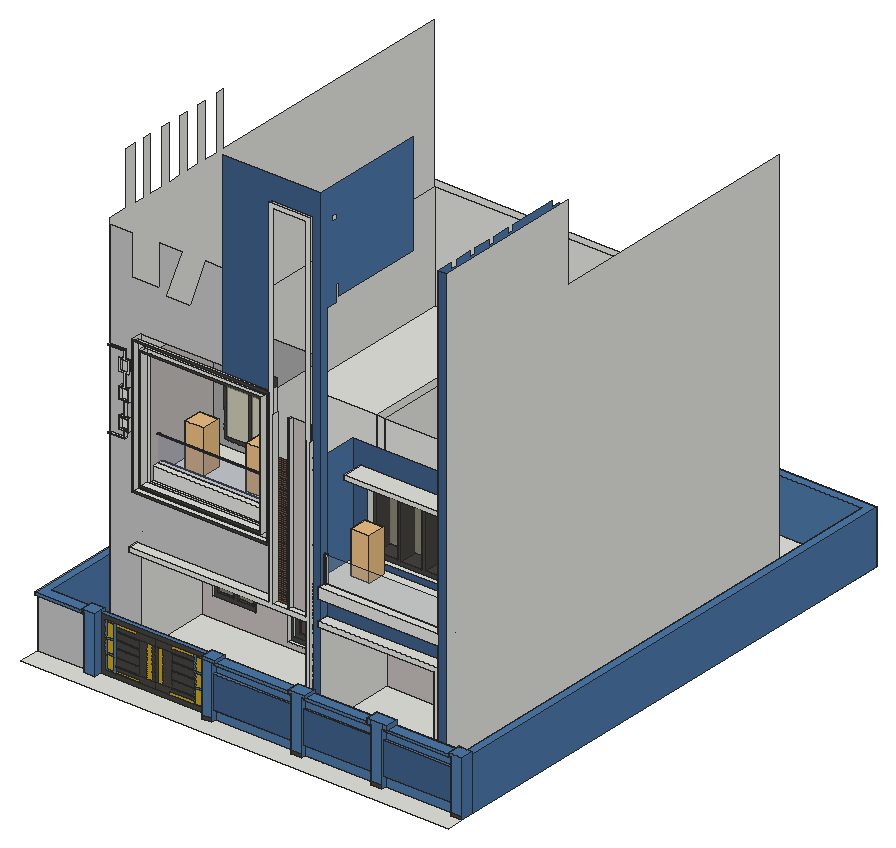
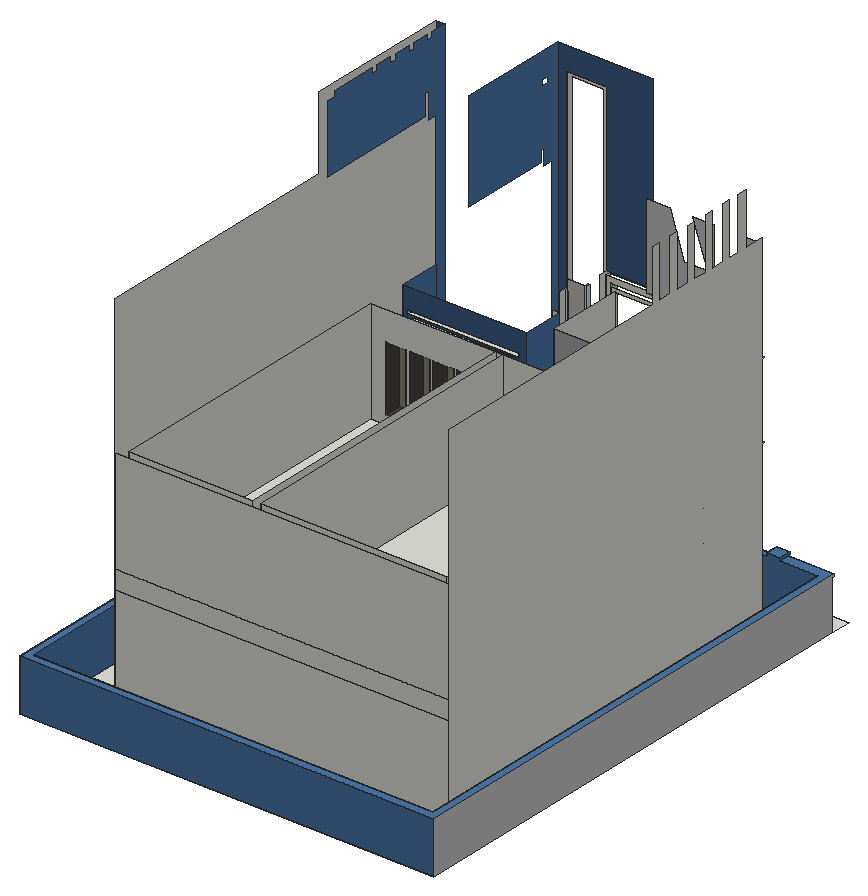
# SketchUp Ruby script. Lengths in inches.
U = 1.inch
M = Sketchup.active_model
def pt(a) = Geom::Point3d.new(a.map { |v| v * U })
def face(e, loops, mat)
  f = e.add_face(loops[0].map { |a| pt(a) })
  loops[1..].each { |l| e.add_face(l.map { |a| pt(a) }).erase! }
  f.material = f.back_material = mat if mat
  f
end
# faces: each face lists its corners as indices into pts; further lists are holes
def faces(e, pts, list, mat = nil) = list.each { |f| face(e, (f[0].is_a?(Array) ? f : [f]).map { |l| l.map { |i| pts[i] } }, mat) }
# xy, xz, yz: faces in a plane at the given z, y or x. An outline is a flat list of corners, or four numbers for a rectangle; further outlines are holes
def ring(l) = l.size == 4 ? [[l[0], l[1]], [l[2], l[1]], [l[2], l[3]], [l[0], l[3]]] : l.each_slice(2).to_a
def flat(e, list, mat, &to3) = list.each { |f| face(e, (f[0].is_a?(Array) ? f : [f]).map { |l| ring(l).map { |u, v| to3.(u, v) } }, mat) }
def xy(e, z, list, mat = nil) = flat(e, list, mat) { |x, y| [x, y, z] }
def xz(e, y, list, mat = nil) = flat(e, list, mat) { |x, z| [x, y, z] }
def yz(e, x, list, mat = nil) = flat(e, list, mat) { |y, z| [x, y, z] }
def lines(e, pts, list) = list.each { |a, b| e.add_line(pt(pts[a]), pt(pts[b])) }
# prism: a flat outline (further loops are holes) pulled along v
def prism(e, loops, v, mat = nil)
  f = face(e, loops, mat); d = Geom::Vector3d.new(v.map { |x| x * U })
  f.pushpull(f.normal.samedirection?(d) ? d.length : -d.length)
end
def box(e, o, s, mat = nil) = prism(e, [[o, [o[0] + s[0], o[1], o[2]], [o[0] + s[0], o[1] + s[1], o[2]], [o[0], o[1] + s[1], o[2]]]], [0, 0, s[2]], mat)
def at(x, y, z, deg = 0) = Geom::Transformation.translation(pt([x, y, z])) * Geom::Transformation.rotation(ORIGIN, Z_AXIS, deg.degrees)
def axes(o, x, y, z) = Geom::Transformation.new([*x, 0, *y, 0, *z, 0, *pt(o).to_a, 1])
def part(name) = M.definitions.add(name)
# library, detail: a bought-in or finely detailed component or shape, given as its bounding box
def library(name, o, s) = part(name).tap { |d| box(d.entities, o, s) }
def detail(e, o, s) = box(e.add_group.entities, o, s)
def put(e, d, t, mat = nil) = e.add_instance(d, t).tap { |i| i.material = mat if mat }
def group(e, t, mat = nil) = e.add_group.tap { |g| g.transformation = t; g.material = mat if mat }.entities
root = M.entities
M.materials.add("!长灌木1").color = [90, 107, 61]
M.materials.add("Brick_09_1K").color = [77, 120, 168]
M.materials.add("Brick_09_1K1").color = [62, 96, 135]
M.materials.add("Glass_Basic_01").color = [161, 173, 186]
M.materials["Glass_Basic_01"].alpha = 0.25
M.materials.add("Glass_Mirror_01").color = [188, 186, 154]
M.materials["Glass_Mirror_01"].alpha = 0.57
M.materials.add("Glass_Sky Reflection_01").color = [126, 138, 183]
M.materials["Glass_Sky Reflection_01"].alpha = 0.25
M.materials.add("Image3").color = [196, 190, 186]
M.materials.add("M02_Ash_Whisper").color = [196, 196, 196]
M.materials.add("M03_Pewter_Shine").color = [168, 168, 168]
M.materials.add("Material20").color = [184, 138, 65]
M.materials.add("Material48").color = [126, 124, 110]
M.materials.add("Metal_32_1K").color = [117, 124, 125]
M.materials.add("Metal_Perforated_08_1K").color = [201, 163, 22]
M.materials.add("Wood_Floor_12_1K").color = [92, 75, 65]
M.materials.add("Wood_Planks_01_1K").color = [69, 67, 63]
M.materials.add("Wood_Veneer_15_1K").color = [132, 88, 57]
c1 = part("组\#1")
xy(c1.entities,0,[[0,0,2.36,2.36],[29.92,0,32.28,2.36],[0,29.92,2.36,32.28],[29.92,29.92,32.28,32.28]],"Material48")
xy(c1.entities,1.57,[[2.36,0.39,2.36,2.36,0.39,2.36,0.39,29.92,2.36,29.92,2.36,31.89,29.92,31.89,29.92,29.92,31.89,29.92,31.89,2.36,29.92,2.36,29.92,0.39]],"Material48")
xy(c1.entities,2.76,[[3.54,0.39,28.74,1.57],[0.39,3.54,1.57,28.74],[30.71,3.54,31.89,28.74],[3.54,30.71,28.74,31.89]],"Material20")
xy(c1.entities,20.08,[[3.54,0.39,28.74,1.57],[0.39,3.54,1.57,28.74],[30.71,3.54,31.89,28.74],[3.54,30.71,28.74,31.89]],"Material20")
xy(c1.entities,21.0625,[[2.36,2.36,29.92,29.92]],"!长灌木1")
xy(c1.entities,21.26,[[2.36,0.39,29.92,2.36],[0.39,2.36,2.36,29.92],[29.92,2.36,31.89,29.92],[2.36,29.92,29.92,31.89]],"Material20")
xy(c1.entities,21.38,[[2.36,2.36,29.92,29.92]],"!长灌木1")
xy(c1.entities,22.83,[[0,0,2.36,2.36],[29.92,0,32.28,2.36],[0,29.92,2.36,32.28],[29.92,29.92,32.28,32.28]],"Material20")
xz(c1.entities,0,[[0,0,2.36,22.83],[29.92,0,32.28,22.83]],"Material20")
xz(c1.entities,0.39,[[[2.36,1.57,29.92,21.26],[3.54,2.76,28.74,20.08]]],"Material20")
xz(c1.entities,1.57,[[3.54,2.76,28.74,20.08]],"Material20")
xz(c1.entities,2.36,[[2.36,21.0625,29.92,21.38],[2.36,21.26,29.92,23.43]],"!长灌木1")
xz(c1.entities,2.36,[[0,0,0,22.83,2.36,22.83,2.36,21.26,0.39,21.26,0.39,1.57,2.36,1.57,2.36,0],[29.92,0,29.92,1.57,31.89,1.57,31.89,21.26,29.92,21.26,29.92,22.83,32.28,22.83,32.28,0]],"Material20")
xz(c1.entities,3.54,[[0.39,2.76,1.57,20.08],[30.71,2.76,31.89,20.08]],"Material20")
xz(c1.entities,28.74,[[0.39,2.76,1.57,20.08],[30.71,2.76,31.89,20.08]],"Material20")
xz(c1.entities,29.92,[[2.36,21.0625,29.92,21.38],[2.36,21.26,29.92,23.43]],"!长灌木1")
xz(c1.entities,29.92,[[0,0,2.36,0,2.36,1.57,0.39,1.57,0.39,22.83,0,22.83],[29.92,0,32.28,0,32.28,22.83,31.89,22.83,31.89,1.57,29.92,1.57],[0.39,21.26,2.36,22.83],[29.92,21.26,31.89,22.83]],"Material20")
xz(c1.entities,30.71,[[3.54,2.76,28.74,20.08]],"Material20")
xz(c1.entities,31.89,[[[2.36,1.57,29.92,21.26],[3.54,2.76,28.74,20.08]]],"Material20")
xz(c1.entities,32.28,[[0,0,2.36,22.83],[29.92,0,32.28,22.83]],"Material20")
yz(c1.entities,0,[[0,0,2.36,22.83],[29.92,0,32.28,22.83]],"Material20")
yz(c1.entities,0.39,[[[2.36,1.57,29.92,21.26],[3.54,2.76,28.74,20.08]]],"Material20")
yz(c1.entities,1.57,[[3.54,2.76,28.74,20.08]],"Material20")
yz(c1.entities,2.36,[[0,0,2.36,0,2.36,1.57,0.39,1.57,0.39,22.83,0,22.83]])
yz(c1.entities,2.36,[[2.36,21.0625,29.92,21.38],[2.36,21.26,29.92,23.43]],"!长灌木1")
yz(c1.entities,2.36,[[29.92,0,32.28,0,32.28,22.83,29.92,22.83,29.92,21.26,31.89,21.26,31.89,1.57,29.92,1.57],[0.39,21.26,2.36,22.83]],"Material20")
yz(c1.entities,3.54,[[0.39,2.76,1.57,20.08],[30.71,2.76,31.89,20.08]],"Material20")
yz(c1.entities,28.74,[[0.39,2.76,1.57,20.08],[30.71,2.76,31.89,20.08]],"Material20")
yz(c1.entities,29.92,[[2.36,21.0625,29.92,21.38],[2.36,21.26,29.92,23.43]],"!长灌木1")
yz(c1.entities,29.92,[[0,0,0,22.83,2.36,22.83,2.36,21.26,0.39,21.26,0.39,1.57,2.36,1.57,2.36,0],[29.92,0,29.92,1.57,31.89,1.57,31.89,21.26,29.92,21.26,29.92,22.83,32.28,22.83,32.28,0]],"Material20")
yz(c1.entities,30.71,[[3.54,2.76,28.74,20.08]],"Material20")
yz(c1.entities,31.89,[[[2.36,1.57,29.92,21.26],[3.54,2.76,28.74,20.08]]],"Material20")
yz(c1.entities,32.28,[[0,0,2.36,22.83],[29.92,0,32.28,22.83]],"Material20")
c2 = part("组\#2")
put(c2.entities,c1,at(24.1,23.99,0))
c3 = part("Potted tree")
put(c3.entities,c2,at(-24.1,-23.99,-1.57))
c4 = library("Group_2",[-1.28,-0.39,0],[21.22,20.51,48.44])
xy(root,0,[[0,0,480,0,480,19,468,19,468,24,390.18,24,390.18,19,378.18,19,378.18,24,300.36,24,300.36,19,288.36,19,288.36,24,199.54,24,199.54,19,188.41,19,188.41,27.57,68.53,27.57,68.53,19,56.53,19,56.53,24,0,24],[[56.53,19,68.53,19,68.53,27.57,188.41,27.57,188.41,19,199.54,19,199.54,24,288.36,24,288.36,19,300.36,19,300.36,24,378.18,24,378.18,19,390.18,19,390.18,24,468,24,468,19,480,19,480,600,0,600,0,24,56.53,24],[9,33,471,591]],[[9,33,471,591],[265,69,265,81,270,81,270,165,71.88,165,71.88,81,36,81,36,534,423,534,423,69,408.87,69,408.87,165,279,165,279,72.06,270,72.06,270,69]],[413,69,423,165],[270,72.06,279,165],
  [36,81,71.88,165],[45,174,261,525],[270,174,414,525]])
xy(root,6,[[168,165,240,168.66]])
xy(root,10,[[172,168.66,204,170.16],[204,168.66,236,170.99]])
xy(root,12,[[199.54,21,288.36,24],[300.36,21,378.18,24],[390.18,21,468,24]],"Brick_09_1K")
xy(root,15,[[177,170.16,199,172.08],[209,170.99,231,172.5],[177,172.08,199,174],[209,172.5,231,174]],"Wood_Planks_01_1K")
xy(root,21.3,[[341,165,401,167.38]])
xy(root,21.88,[[84,165,132,166.72]])
xy(root,25.3,[[345,167.38,369,167.38,373,167.86,373,170.69,345,170.69],[373,167.38,397,167.38,397,170.69,373,167.86],[373,167.86,397,170.69,373,170.69],[345,170.69,373,170.69,373,173.53,369,174,345,174],[373,170.69,397,170.69,373,173.53],
  [397,170.69,397,174,373,174,373,173.53]],"Wood_Planks_01_1K")
xy(root,25.88,[[88,166.72,106,170.36],[110,166.72,128,170.36],[88,170.36,106,174],[110,170.36,128,174]],"Wood_Planks_01_1K")
xy(root,48,[[199.54,21,288.36,24],[300.36,21,378.18,24],[390.18,21,468,24]],"Brick_09_1K")
xy(root,57,[[0,21,56.53,24],[199.54,21,288.36,24],[300.36,21,378.18,24],[390.18,21,468,24]],"Brick_09_1K")
xy(root,60,[[53.53,19,56.53,21],[199.54,19,202.54,21],[285.36,19,288.36,21],[300.36,19,303.36,21],[373.51,19,378.18,21],
  [390.18,19,395.5625,21],[465,19,468,21],[0,21,53.53,21,53.53,33,9,33,9,591,471,591,471,33,480,33,480,600,0,600],[202.54,21,285.36,33],[303.36,21,373.51,33],
  [395.5625,21,465,33],[68.53,27.57,188.41,33]],"Brick_09_1K")
xy(root,63,[[53.53,19,68.53,33],[188.41,19,202.54,33],[285.36,19,303.36,33],[465,19,480,33]],"Brick_09_1K")
xy(root,65.38,[[373.51,19,395.5625,33]],"Brick_09_1K")
xy(root,81,[[177,170.16,199,172.08],[209,170.99,231,172.5],[177,172.08,199,174],[209,172.5,231,174]],"Wood_Planks_01_1K")
xy(root,86,[[172,168.66,204,170.16],[204,168.66,236,170.99]])
xy(root,86,[[88,166.72,106,170.36],[110,166.72,128,170.36],[345,167.38,345,170.69,373,170.69,373,167.86,369,167.38],[373,167.38,373,167.86,397,170.69,397,167.38],[373,167.86,373,170.69,397,170.69],
  [88,170.36,106,174],[110,170.36,128,174],[345,170.69,345,174,369,174,373,173.53,373,170.69],[373,170.69,373,173.53,397,170.69],[397,170.69,373,173.53,373,174,397,174]],"Wood_Planks_01_1K")
xy(root,90,[[84,165,132,166.72],[168,165,240,168.66],[341,165,401,167.38]])
xy(root,102,[[66.12,69,71.88,81],[71.88,69,71.88,165,261,165,261,81,223.07,81,223.07,69],[223.07,69,265,81],[279,69,408.87,165],[261,81,270,165],
  [270,81,279,165]])
xy(root,107,[[66.12,69,223.07,81],[228.07,69,265,69,265,75.9,244.4,75.9,244.4,72.3125,242.32,72.3125,242.32,75.9,228.07,75.9]])
xy(root,108,[[279,69,413,81]])
xy(root,130,[[279,69,413,81]])
xy(root,142,[[279,69,413,69,413,77.38,282.2,77.38,282.2,76.04,279,76.04],[282.2,77.38,413,77.38,413,129,270,129,270,81,279,81,279,78.72,282.2,78.72],[261,81,270,165],[45,174,261,525],[270,174,414,525]])
xy(root,148,[[287,129,401,135.39]])
xy(root,152,[[291,135.39,314.5,154.7],[318.5,135.39,342,174],[346,135.39,369.5,174],[373.5,135.39,397,174],[291,154.7,314.5,174]],"Wood_Planks_01_1K")
xy(root,164,[[70,69,223.07,81]])
xy(root,166,[[72,69,221.07,75]])
xy(root,172,[[78,69,215.07,75],[279,76.04,282.2,78.72]])
xy(root,174,[[80,69,213.07,77.68]])
xy(root,175.72,[[84,77.68,209.07,81]])
xy(root,178,[[84,93.35,209.07,165]])
xy(root,190,[[84,81,209.07,81,209.07,87.18,84,87.26],[209.07,87.18,209.07,93.35,84,93.35,84,87.26]])
xy(root,207.65,[[36,78,55,81]])
xy(root,208.65,[[36,78,54,81]])
xy(root,215.87,[[48.51,78,54,81],[55,78,59.4,81]])
xy(root,216.87,[[49.51,78,58.4,81]])
xy(root,228,[[291,135.39,314.5,154.7],[318.5,135.39,342,174],[346,135.39,369.5,174],[373.5,135.39,397,174],[291,154.7,314.5,174]],"Wood_Planks_01_1K")
xy(root,228.74,[[49.51,78,58.4,81]])
xy(root,229.74,[[48.51,78,54,81],[55,78,59.4,81]])
xy(root,232,[[287,129,401,135.39]])
xy(root,233.78,[[279.03,105,407.71,129]])
xy(root,238.38,[[279.03,105,407.71,129]])
xy(root,245.55,[[48.51,78,54,81],[55,78,59.4,81]])
xy(root,246.55,[[49.51,78,58.4,81]])
xz(root,19,[[56.53,0,68.53,63],[188.41,4,199.54,60],[288.36,4,300.36,4,300.36,60,303.36,60,303.36,63,285.36,63,285.36,60,288.36,60],[378.18,4,390.18,65.38],[468,4,480,4,480,63,465,63,465,60,468,60],
  [53.53,60,56.53,63],[188.41,60,202.54,63],[373.51,60,378.18,65.38],[390.18,60,395.5625,65.38]],"Brick_09_1K")
xz(root,19,[[188.41,0,199.54,4],[288.36,0,300.36,4],[378.18,0,390.18,4],[468,0,480,4]],"Wood_Planks_01_1K")
xz(root,21,[[0,57,56.53,60],[199.54,57,288.36,60],[300.36,57,378.18,60],[390.18,57,468,60]],"Brick_09_1K")
xz(root,21,[[199.54,12,288.36,48],[300.36,12,378.18,48],[390.18,12,468,48]],"Brick_09_1K1")
xz(root,24,[[199.54,0,288.36,12],[300.36,0,378.18,12],[390.18,0,468,12],[199.54,48,288.36,57],[300.36,48,378.18,57],
  [390.18,48,468,57]],"Brick_09_1K")
xz(root,24,[[0,0,56.53,57]],"M02_Ash_Whisper")
xz(root,27.57,[[[72.53,4,84.53,56],[74.53,6,82.53,54]],[[172.41,4,184.41,56],[174.41,6,182.41,54]],[84.53,12,110.66,13],[147.49,12,172.41,13],[84.53,20.75,110.66,21.75],
  [147.49,20.75,172.41,21.75],[74.53,21.33,82.53,23.33],[174.41,21.33,182.41,23.33],[84.53,29.5,110.66,30.5],[147.49,29.5,172.41,30.5],
  [74.53,36.67,82.53,38.67],[174.41,36.67,182.41,38.67],[84.53,38.25,110.66,39.25],[147.49,38.25,172.41,39.25],[84.53,47,110.66,48],
  [147.49,47,172.41,48]],"Brick_09_1K")
xz(root,27.57,[[84.53,5.11,111.61,8],[145.17,5.11,172.41,8],[74.53,6,82.53,21.33],[174.41,6,182.41,21.33],[119.57,12,125.31,48],
  [131.65,12,137.98,48],[74.53,23.33,82.53,36.67],[174.41,23.33,182.41,36.67],[74.53,38.67,82.53,54],[174.41,38.67,182.41,54],
  [84.53,52,108.53,56],[148.41,52,172.41,56]],"Metal_Perforated_08_1K")
xz(root,27.57,[[[68.53,0,188.41,60],[72.53,4,184.41,56]],[84.53,4,128.47,4,128.47,12,84.53,12,84.53,8,111.61,8,111.61,5.11,84.53,5.11],[128.47,4,172.41,4,172.41,5.11,145.17,5.11,145.17,8,172.41,8,172.41,12,128.47,12],[110.66,12,119.57,48],[125.31,12,128.47,48],
  [128.47,12,131.65,48],[137.98,12,147.49,48],[84.53,13,110.66,20.75],[147.49,13,172.41,20.75],[84.53,21.75,110.66,29.5],
  [147.49,21.75,172.41,29.5],[84.53,30.5,110.66,38.25],[147.49,30.5,172.41,38.25],[84.53,39.25,110.66,47],[147.49,39.25,172.41,47],
  [84.53,48,128.47,48,128.47,56,108.53,56,108.53,52,84.53,52],[128.47,48,172.41,48,172.41,52,148.41,52,148.41,56,128.47,56]],"Wood_Planks_01_1K")
xz(root,33,[[9,0,9,60,53.53,60,53.53,63,68.53,63,68.53,60,188.41,60,188.41,63,202.54,63,202.54,60,285.36,60,285.36,63,303.36,63,303.36,60,373.51,60,373.51,65.38,395.5625,65.38,395.5625,60,465,60,465,63,471,63,471,0],[471,60,480,63]],"Brick_09_1K")
xz(root,69,[[[265,0,270,0,270,509.43,223.07,509.43,223.07,107,66.12,107,66.12,102,265,102],[228.07,107,265,504.43]],[408.87,0,413,0,413,108,279,108,279,102,408.87,102],[279,130,413,142]])
xz(root,69,[[413,0,423,506.58]],"Brick_09_1K1")
xz(root,69,[[[70,164,223.07,318],[72,166,221.07,316]],[[78,172,215.07,310],[80,174,213.07,308]]],"Wood_Planks_01_1K")
xz(root,72.06,[[270,0,279,0,279,536.58,169.4,536.58,169.4,318,223.07,318,223.07,509.43,270,509.43]],"Brick_09_1K1")
xz(root,72.3125,[[242.32,107,244.4,297.09]])
xz(root,75,[[[72,166,221.07,316],[78,172,215.07,310]]])
xz(root,75.9,[[244.4,107,265,297.09]],"Image3")
xz(root,75.9,[[228.07,107,242.32,108.9],[228.07,108.9,242.32,110.8],[228.07,110.8,242.32,112.7],[228.07,112.7,242.32,114.6],[228.07,114.6,242.32,116.5],
  [228.07,116.5,242.32,118.41],[228.07,118.41,242.32,120.31],[228.07,120.31,242.32,122.21],[228.07,122.21,242.32,124.11],[228.07,124.11,242.32,126.01],
  [228.07,126.01,242.32,127.91],[228.07,127.91,242.32,129.8125],[228.07,129.8125,242.32,131.71],[228.07,131.71,242.32,133.61],[228.07,133.61,242.32,135.51],
  [228.07,135.51,242.32,137.42],[228.07,137.42,242.32,139.32],[228.07,139.32,242.32,141.22],[228.07,141.22,242.32,143.12],[228.07,143.12,242.32,145.02],
  [228.07,145.02,242.32,146.92],[228.07,146.92,242.32,148.82],[228.07,148.82,242.32,150.72],[228.07,150.72,242.32,152.62],[228.07,152.62,242.32,154.52],
  [228.07,154.52,242.32,156.42],[228.07,156.42,242.32,158.33],[228.07,158.33,242.32,160.23],[228.07,160.23,242.32,162.13],[228.07,162.13,242.32,164.03],
  [228.07,164.03,242.32,165.93],[228.07,165.93,242.32,167.83],[228.07,167.83,242.32,169.73],[228.07,169.73,242.32,171.63],[228.07,171.63,242.32,173.53],
  [228.07,173.53,242.32,175.43],[228.07,175.43,242.32,177.33],[228.07,177.33,242.32,179.24],[228.07,179.24,242.32,181.14],[228.07,181.14,242.32,183.04],
  [228.07,183.04,242.32,184.9375],[228.07,184.9375,242.32,186.84],[228.07,186.84,242.32,188.74],[228.07,188.74,242.32,190.64],[228.07,190.64,242.32,192.54],
  [228.07,192.54,242.32,194.44],[228.07,194.44,242.32,196.34],[228.07,196.34,242.32,198.25],[228.07,198.25,242.32,200.15],[228.07,200.15,242.32,202.05],
  [228.07,202.05,242.32,203.95],[228.07,203.95,242.32,205.85],[228.07,205.85,242.32,207.75],[228.07,207.75,242.32,209.65],[228.07,209.65,242.32,211.55],
  [228.07,211.55,242.32,213.45],[228.07,213.45,242.32,215.35],[228.07,215.35,242.32,217.25],[228.07,217.25,242.32,219.16],[228.07,219.16,242.32,221.06],
  [228.07,221.06,242.32,222.96],[228.07,222.96,242.32,224.86],[228.07,224.86,242.32,226.76],[228.07,226.76,242.32,228.66],[228.07,228.66,242.32,230.5625],
  [228.07,230.5625,242.32,232.46],[228.07,232.46,242.32,234.36],[228.07,234.36,242.32,236.26],[228.07,236.26,242.32,238.17],[228.07,238.17,242.32,240.07],
  [228.07,240.07,242.32,241.97],[228.07,241.97,242.32,243.87],[228.07,243.87,242.32,245.77],[228.07,245.77,242.32,247.67],[228.07,247.67,242.32,249.57],
  [228.07,249.57,242.32,251.47]],"Wood_Veneer_15_1K")
xz(root,76.04,[[279,142,282.2,172]],"Metal_32_1K")
xz(root,77.38,[[282.2,142,413,172]],"Glass_Basic_01")
xz(root,77.68,[[[80,174,213.07,308],[84,175.72,209.07,304]]])
xz(root,78,[[[36,207.65,55,207.65,55,215.87,59.4,215.87,59.4,229.74,55,229.74,55,245.55,59.4,245.55,59.4,259.42,55,259.42,55,274.21,59.4,274.21,59.4,288.08,55,288.08,55,296.99,36,296.99,36,295.99,54,295.99,54,288.08,48.51,288.08,48.51,274.21,54,274.21,54,259.42,48.51,259.42,48.51,245.55,54,245.55,54,229.74,48.51,229.74,48.51,215.87,54,215.87,54,208.65,36,208.65],[49.51,216.87,58.4,228.74],[49.51,246.55,58.4,258.42],[49.51,275.21,58.4,287.08]]])
xz(root,78.72,[[279,142,282.2,172]])
xz(root,81,[[265,0,270,102],[223.07,102,261,120],[270,102,279,142],[223.07,142,261,178],[270,142,279,262],
  [84,175.72,209.07,190],[49.51,216.87,58.4,228.74],[49.51,246.55,58.4,258.42]])
xz(root,81,[[279,108,413,130]],"Brick_09_1K1")
xz(root,81,[[36,0,71.88,0,71.88,102,66.12,102,66.12,107,223.07,107,223.07,164,70,164,70,318,169.4,318,169.4,415.99,142.82,415.99,126.42,365.83,98.85,365.83,116.24,415.99,91.1,415.99,91.1,371.59,60.8,371.59,60.8,415.99,36,415.99,36,296.99,55,296.99,55,288.08,59.4,288.08,59.4,274.21,55,274.21,55,259.42,59.4,259.42,59.4,245.55,55,245.55,55,229.74,59.4,229.74,59.4,215.87,55,215.87,55,207.65,36,207.65],[36,208.65,54,208.65,54,215.87,48.51,215.87,48.51,229.74,54,229.74,54,245.55,48.51,245.55,48.51,259.42,54,259.42,54,274.21,48.51,274.21,48.51,288.08,54,288.08,54,295.99,36,295.99]],"M02_Ash_Whisper")
xz(root,93.35,[[84,178,209.07,190]])
xz(root,105,[[279.03,233.78,407.71,238.38]])
xz(root,129,[[[270,142,413,262],[287,148,401,232],[279.03,233.78,407.71,238.38]]],"Brick_09_1K1")
xz(root,135.39,[[[287,148,401,232],[373.5,152,397,228],[346,152,369.5,228],[318.5,152,342,228],[291,152,314.5,228]]],"Wood_Planks_01_1K")
xz(root,154.7,[[291,152,314.5,228],[317.38,152,340.88,228],[344.88,152,368.38,228],[372.83,152,396.33,228]],"Glass_Mirror_01")
xz(root,165,[[408.87,0,413,0,413,120,270,120,270,102,408.87,102],[71.88,102,261,120]])
xz(root,165,[[100,188,124,264],[128,188,152,264]],"Glass_Mirror_01")
xz(root,165,[[[71.88,0,270,102],[168,6,240,90],[84,21.88,132,90]],[[279,0,408.87,102],[341,21.3,401,90]]],"Image3")
xz(root,165,[[[84,178,209.07,304],[96,184,156,268],[174,184,204,268]]],"M03_Pewter_Shine")
xz(root,165,[[[96,184,156,268],[100,188,124,264],[128,188,152,264]],[[174,184,204,268],[177,187,201,265]],[177,187,201,265]],"Wood_Planks_01_1K")
xz(root,166.72,[[[84,21.88,132,90],[88,25.88,106,86],[110,25.88,128,86]]],"Wood_Planks_01_1K")
xz(root,167.38,[[[341,21.3,401,90],[345,25.3,369,86],[373,25.3,397,86]]],"Wood_Planks_01_1K")
xz(root,168.66,[[[168,6,240,90],[172,10,236,86]]],"Wood_Planks_01_1K")
xz(root,170.16,[[[172,10,204,86],[177,15,199,81]]],"Wood_Planks_01_1K")
xz(root,170.36,[[88,25.88,106,86],[110,25.88,128,86]],"Glass_Mirror_01")
xz(root,170.69,[[345,25.3,369,86],[369,25.3,397,86]],"Glass_Mirror_01")
xz(root,170.99,[[[204,10,236,86],[209,15,231,81]]],"Wood_Planks_01_1K")
xz(root,172.08,[[177,15,199,81]],"Wood_Floor_12_1K")
xz(root,172.5,[[209,15,231,81]],"Wood_Floor_12_1K")
xz(root,174,[[[45,0,261,120],[209,15,231,81],[177,15,199,81],[88,25.88,106,86],[110,25.88,128,86]],[261,0,270,120],[[270,0,414,120],[345,25.3,369,86],[373,25.3,397,86]],[45,142,261,262],[261,142,270,262],
  [[270,142,414,262],[291,152,314.5,228],[318.5,152,342,228],[346,152,369.5,228],[373.5,152,397,228]]])
xz(root,525,[[45,0,261,120],[270,0,414,120],[45,142,261,262],[270,142,414,262]])
xz(root,534,[[36,0,423,120],[36,120,423,142],[36,142,423,262]])
xz(root,591,[[9,0,471,60]],"Brick_09_1K")
xz(root,600,[[0,0,480,60]],"Brick_09_1K")
yz(root,0,[[24,0,24,57,21,57,21,60,600,60,600,0]],"M02_Ash_Whisper")
yz(root,9,[[33,0,591,60]],"Brick_09_1K")
yz(root,36,[[81,0,81,207.65,78,207.65,78,208.65,81,208.65,81,295.99,78,295.99,78,296.99,81,296.99,81,421.99,103.39,421.99,103.39,481.99,115.39,481.99,115.39,421.99,127.86,421.99,127.86,481.99,137,481.99,137,421.99,153.33,421.99,153.33,481.99,162.48,481.99,162.48,421.99,178.8125,421.99,178.8125,481.99,187.95,481.99,187.95,421.99,204.29,421.99,204.29,481.99,213.43,481.99,213.43,421.99,229.77,421.99,229.77,481.99,238.91,481.99,238.91,421.99,534,421.99,534,0]])
yz(root,45,[[174,0,525,120],[174,142,525,262]])
yz(root,48.51,[[78,215.87,81,229.74],[78,245.55,81,259.42]])
yz(root,49.51,[[78,216.87,81,228.74],[78,246.55,81,258.42]])
yz(root,53.53,[[19,60,33,63]],"Brick_09_1K")
yz(root,54,[[78,208.65,81,215.87],[78,229.74,81,245.55]])
yz(root,55,[[78,207.65,81,208.65],[78,208.65,81,215.87],[78,229.74,81,245.55]])
yz(root,56.53,[[19,0,19,60,21,60,21,57,24,57,24,0]],"Brick_09_1K")
yz(root,58.4,[[78,216.87,81,228.74],[78,246.55,81,258.42]])
yz(root,59.4,[[78,215.87,81,229.74],[78,245.55,81,259.42]])
yz(root,66.12,[[69,102,81,107]])
yz(root,68.53,[[19,0,27.57,63],[27.57,60,33,63]],"Brick_09_1K")
yz(root,70,[[69,164,81,318]])
yz(root,71.88,[[81,0,165,102]])
yz(root,72,[[69,166,75,316]])
yz(root,78,[[69,172,75,310]])
yz(root,80,[[69,174,77.68,308]])
yz(root,84,[[165,21.88,166.72,90]])
yz(root,84,[[[77.68,175.72,81,175.72,81,190,93.35,190,93.35,178,165,178,165,304,77.68,304],[87.18,219.28,87.02,219.3,86.87,219.36,86.74,219.46,86.64,219.59,86.58,219.74,86.55,219.9,86.58,220.06,86.64,220.21,86.74,220.34,86.87,220.43,87.02,220.5,87.18,220.52,87.34,220.5,87.49,220.43,87.62,220.34,87.71,220.21,87.78,220.06,87.8,219.9,87.78,219.74,87.71,219.59,87.62,219.46,87.49,219.36,87.34,219.3]]],"Image3")
yz(root,88,[[166.72,25.88,170.36,86],[170.36,25.88,174,86]],"Wood_Planks_01_1K")
yz(root,106,[[166.72,25.88,170.36,86],[170.36,25.88,174,86]],"Wood_Planks_01_1K")
yz(root,110,[[166.72,25.88,170.36,86],[170.36,25.88,174,86]],"Wood_Planks_01_1K")
yz(root,128,[[166.72,25.88,170.36,86],[170.36,25.88,174,86]],"Wood_Planks_01_1K")
yz(root,132,[[165,21.88,166.72,90]])
yz(root,168,[[165,6,168.66,90]])
yz(root,172,[[168.66,10,170.16,86]])
yz(root,177,[[170.16,15,172.08,81],[172.08,15,174,81]],"Wood_Planks_01_1K")
yz(root,188.41,[[19,0,27.57,63],[27.57,60,33,63]],"Brick_09_1K")
yz(root,199,[[170.16,15,172.08,81],[172.08,15,174,81]],"Wood_Planks_01_1K")
yz(root,199.54,[[19,0,24,0,24,12,21,12,21,48,24,48,24,57,21,57,21,60,19,60]],"Brick_09_1K")
yz(root,202.54,[[19,60,33,63]],"Brick_09_1K")
yz(root,204,[[170.16,10,170.99,86]])
yz(root,209,[[170.99,15,172.5,81],[172.5,15,174,81]],"Wood_Planks_01_1K")
yz(root,209.07,[[77.68,175.72,77.68,304,165,304,165,178,93.35,178,93.35,190,87.18,190,87.18,219.27,87.34,219.3,87.49,219.36,87.62,219.46,87.71,219.59,87.78,219.74,87.8,219.9,87.78,220.06,87.71,220.21,87.62,220.34,87.49,220.44,87.34,220.5,87.18,220.52,87.01,220.5,86.86,220.44,86.74,220.34,86.64,220.21,86.58,220.06,86.55,219.9,86.58,219.74,86.64,219.59,86.74,219.46,86.86,219.36,87.01,219.3,87.18,219.27,87.18,190,81,190,81,175.72]])
yz(root,213.07,[[69,174,77.68,308]])
yz(root,215.07,[[69,172,75,310]])
yz(root,221.07,[[69,166,75,316]])
yz(root,223.07,[[69,107,81,164],[69,164,81,318]])
yz(root,228.07,[[69,107,75.9,297.09]])
yz(root,231,[[170.99,15,172.5,81],[172.5,15,174,81]],"Wood_Planks_01_1K")
yz(root,236,[[168.66,10,170.99,86]])
yz(root,240,[[165,6,168.66,90]])
yz(root,242.32,[[72.3125,107,75.9,297.09]])
yz(root,244.4,[[72.3125,107,75.9,297.09]])
yz(root,261,[[174,0,525,120],[81,102,165,120],[81,142,165,178],[174,142,525,262]])
yz(root,265,[[69,0,81,102],[69,107,75.9,142],[69,142,75.9,284]])
yz(root,270,[[69,0,72.06,284],[72.06,0,81,142],[81,0,165,102],[174,0,525,120],[81,102,165,120],
  [72.06,142,81,284],[174,142,525,262]])
yz(root,270,[[81,142,129,262]],"Brick_09_1K")
yz(root,279,[[72.06,0,165,102],[69,102,72.06,108],[72.06,102,81,108],[69,130,72.06,142],[72.06,130,81,130,81,142,78.72,142,78.72,172,76.04,172,76.04,142,72.06,142]])
yz(root,279,[[72.06,108,81,130],[[72.06,142,76.04,142,76.04,172,78.72,172,78.72,142,81,142,81,416.58,93,416.58,93,434.58,97.45,434.58,97.45,421.99,201,421.99,201,536.58,72.06,536.58],[87.5,500.58,95.04,506.58]]],"Brick_09_1K")
yz(root,279.03,[[105,233.78,129,238.38]])
yz(root,282.2,[[76.04,142,77.38,172],[77.38,142,78.72,172]])
yz(root,285.36,[[19,60,33,63]],"Brick_09_1K")
yz(root,287,[[129,148,135.39,232]])
yz(root,288.36,[[19,0,19,60,21,60,21,57,24,57,24,48,21,48,21,12,24,12,24,0]],"Brick_09_1K")
yz(root,291,[[135.39,152,154.7,228],[154.7,152,174,228]],"Wood_Planks_01_1K")
yz(root,300.36,[[19,0,24,0,24,12,21,12,21,48,24,48,24,57,21,57,21,60,19,60]],"Brick_09_1K")
yz(root,303.36,[[19,60,33,63]],"Brick_09_1K")
yz(root,314.5,[[135.39,152,154.7,228],[154.7,152,174,228]],"Wood_Planks_01_1K")
yz(root,318.5,[[135.39,152,174,228]],"Wood_Planks_01_1K")
yz(root,341,[[165,21.3,167.38,90]])
yz(root,342,[[135.39,152,174,228]],"Wood_Planks_01_1K")
yz(root,345,[[167.38,25.3,170.69,86],[170.69,25.3,174,86]],"Wood_Planks_01_1K")
yz(root,346,[[135.39,152,174,228]],"Wood_Planks_01_1K")
yz(root,369.5,[[135.39,152,174,228]],"Wood_Planks_01_1K")
yz(root,373,[[167.38,25.3,174,86]])
yz(root,373.5,[[135.39,152,174,228]],"Wood_Planks_01_1K")
yz(root,373.51,[[19,60,33,65.38]],"Brick_09_1K")
yz(root,378.18,[[19,0,19,60,21,60,21,57,24,57,24,48,21,48,21,12,24,12,24,0]],"Brick_09_1K")
yz(root,390.18,[[19,0,24,0,24,12,21,12,21,48,24,48,24,57,21,57,21,60,19,60]],"Brick_09_1K")
yz(root,395.5625,[[19,60,33,65.38]],"Brick_09_1K")
yz(root,397,[[167.38,25.3,170.69,86],[170.69,25.3,174,86],[135.39,152,174,228]],"Wood_Planks_01_1K")
yz(root,401,[[165,21.3,167.38,90],[129,148,135.39,152],[129,152,135.39,232]])
yz(root,407.71,[[105,233.78,129,238.38]])
yz(root,408.87,[[69,0,165,102]])
yz(root,413,[[69,0,69,108,81,108,81,117.54,165,117.54,165,0],[81,117.54,165,120]])
yz(root,413,[[69,108,81,130],[69,142,69,506.58,87.5,506.58,87.5,500.58,95.04,500.58,95.04,506.58,113.85,506.58,113.85,500.58,121.39,500.58,121.39,506.58,140.21,506.58,140.21,500.58,147.74,500.58,147.74,506.58,166.56,506.58,166.56,500.58,174.09,500.58,174.09,506.58,228.37,506.58,228.37,500.58,238.37,500.58,238.37,421.99,97.45,421.99,97.45,446.58,92,446.58,92,444.58,92.26,444.58,92.26,416.58,81,416.58,81,142],[81,142,129,262]],"Brick_09_1K")
yz(root,414,[[174,0,525,120],[174,142,525,262]])
yz(root,423,[[69,0,534,0,534,421.99,238.37,421.99,238.37,506.58,69,506.58]])
yz(root,465,[[19,60,33,63]],"Brick_09_1K")
yz(root,468,[[19,0,19,60,21,60,21,57,24,57,24,48,21,48,21,12,24,12,24,0]],"Brick_09_1K")
yz(root,471,[[33,0,591,60]],"Brick_09_1K")
yz(root,480,[[19,0,33,63],[33,0,600,60]],"Brick_09_1K")
p = [[209.07,87.18,219.27],[209.07,87.18,219.33],[83.65,87.26,219.33],[83.65,87.26,190],[84,87.26,190],[209.07,87.18,190],
  [84,87.02,219.3],[209.07,87.01,219.3],[209.07,86.86,219.36],[84,86.87,219.36],[84,87.18,219.28],[84,87.34,219.3],
  [209.07,87.34,219.3],[84,87.49,219.36],[209.07,87.49,219.36],[209.07,86.74,219.46],[84,86.74,219.46],[84,87.62,219.46],
  [209.07,87.62,219.46],[209.07,86.64,219.59],[84,86.64,219.59],[84,87.71,219.59],[209.07,87.71,219.59],[209.07,86.58,219.74],
  [84,86.58,219.74],[84,87.78,219.74],[209.07,87.78,219.74],[209.07,86.55,219.9],[84,86.55,219.9],[84,87.8,219.9],
  [209.07,87.8,219.9],[209.07,86.58,220.06],[84,86.58,220.06],[84,87.78,220.06],[209.07,87.78,220.06],[209.07,86.64,220.21],
  [84,86.64,220.21],[84,87.71,220.21],[209.07,87.71,220.21],[209.07,86.74,220.34],[84,86.74,220.34],[84,87.62,220.34],
  [209.07,87.62,220.34],[209.07,86.86,220.44],[84,86.87,220.43],[84,87.49,220.43],[209.07,87.49,220.44],[209.07,87.01,220.5],
  [84,87.02,220.5],[84,87.34,220.5],[209.07,87.34,220.5],[209.07,87.18,220.52],[84,87.18,220.52],[71.88,165,120],
  [71.88,81,120],[270,174,120],[270,165,120],[36,165,142],[261,165,142],[36,165,178],
  [84,165,178],[209.07,165,178],[261,165,178],[413,81,142],[423,81,142],[188.41,27.57,12],
  [196.41,27.57,12]]
faces(root,p,[[0,1,2,3,4,5]],"Glass_Sky Reflection_01")
faces(root,p,[[6,7,8,9],[10,0,7,6],[11,12,0,10],[13,14,12,11],[9,8,15,16],[17,18,14,13],[15,19,20,16],[17,21,22,18],
  [19,23,24,20],[21,25,26,22],[23,27,28,24],[25,29,30,26],[27,31,32,28],[29,33,34,30],[31,35,36,32],[33,37,38,34],
  [35,39,40,36],[37,41,42,38],[40,39,43,44],[45,46,42,41],[44,43,47,48],[49,50,46,45],[48,47,51,52],[52,51,50,49]])
lines(root,p,[[53,54],[55,56],[57,58],[59,60],[61,62],[63,64],[65,66]])
put(root,c3,at(322.82,33.25,0),"M02_Ash_Whisper")
put(root,c4,at(289.23,103.11,140.27))
put(root,c4,at(163.58,114,177.93))
put(root,c4,at(100.34,107.11,181))
